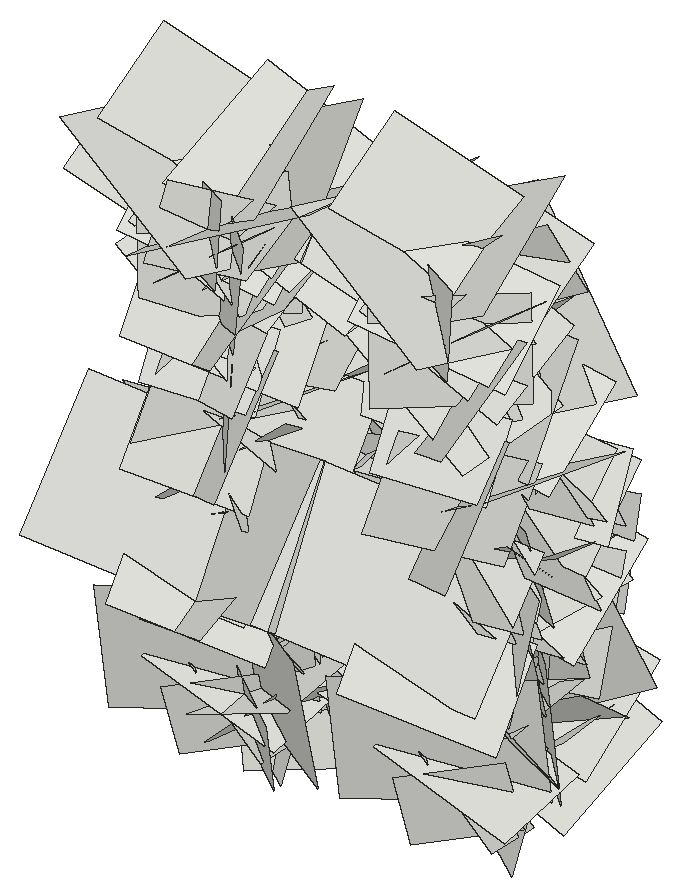
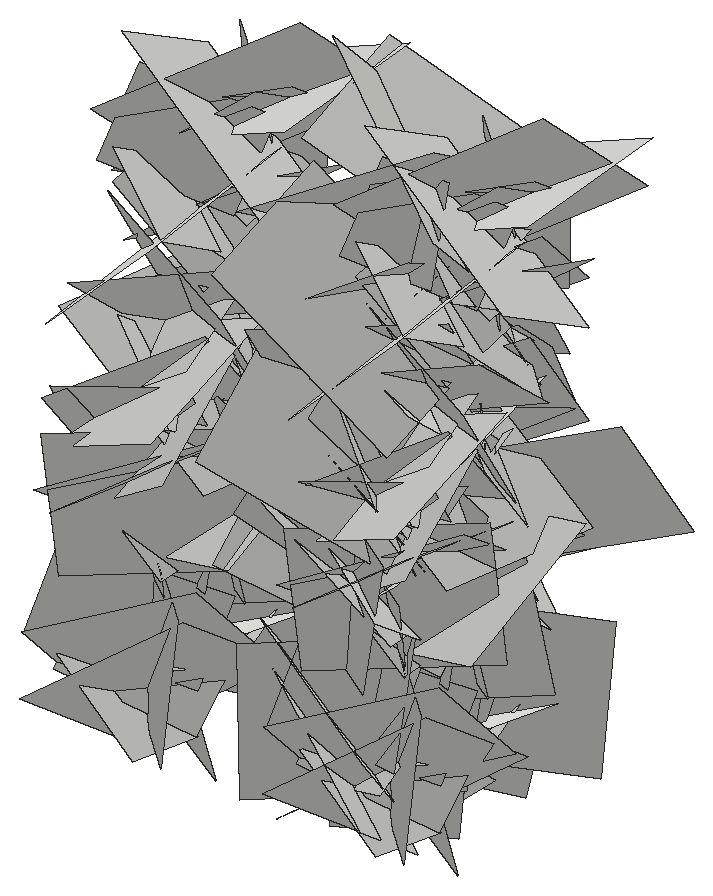
# SketchUp Ruby script. Lengths in inches.
U = 1.inch
M = Sketchup.active_model
def pt(a) = Geom::Point3d.new(a.map { |v| v * U })
def face(e, loops, mat)
  f = e.add_face(loops[0].map { |a| pt(a) })
  loops[1..].each { |l| e.add_face(l.map { |a| pt(a) }).erase! }
  f.material = f.back_material = mat if mat
  f
end
# faces: each face lists its corners as indices into pts; further lists are holes
def faces(e, pts, list, mat = nil) = list.each { |f| face(e, (f[0].is_a?(Array) ? f : [f]).map { |l| l.map { |i| pts[i] } }, mat) }
# xy, xz, yz: faces in a plane at the given z, y or x. An outline is a flat list of corners, or four numbers for a rectangle; further outlines are holes
def ring(l) = l.size == 4 ? [[l[0], l[1]], [l[2], l[1]], [l[2], l[3]], [l[0], l[3]]] : l.each_slice(2).to_a
def flat(e, list, mat, &to3) = list.each { |f| face(e, (f[0].is_a?(Array) ? f : [f]).map { |l| ring(l).map { |u, v| to3.(u, v) } }, mat) }
def xy(e, z, list, mat = nil) = flat(e, list, mat) { |x, y| [x, y, z] }
def xz(e, y, list, mat = nil) = flat(e, list, mat) { |x, z| [x, y, z] }
def yz(e, x, list, mat = nil) = flat(e, list, mat) { |y, z| [x, y, z] }
def lines(e, pts, list) = list.each { |a, b| e.add_line(pt(pts[a]), pt(pts[b])) }
# prism: a flat outline (further loops are holes) pulled along v
def prism(e, loops, v, mat = nil)
  f = face(e, loops, mat); d = Geom::Vector3d.new(v.map { |x| x * U })
  f.pushpull(f.normal.samedirection?(d) ? d.length : -d.length)
end
def box(e, o, s, mat = nil) = prism(e, [[o, [o[0] + s[0], o[1], o[2]], [o[0] + s[0], o[1] + s[1], o[2]], [o[0], o[1] + s[1], o[2]]]], [0, 0, s[2]], mat)
def at(x, y, z, deg = 0) = Geom::Transformation.translation(pt([x, y, z])) * Geom::Transformation.rotation(ORIGIN, Z_AXIS, deg.degrees)
def axes(o, x, y, z) = Geom::Transformation.new([*x, 0, *y, 0, *z, 0, *pt(o).to_a, 1])
def part(name) = M.definitions.add(name)
# library, detail: a bought-in or finely detailed component or shape, given as its bounding box
def library(name, o, s) = part(name).tap { |d| box(d.entities, o, s) }
def detail(e, o, s) = box(e.add_group.entities, o, s)
def put(e, d, t, mat = nil) = e.add_instance(d, t).tap { |i| i.material = mat if mat }
def group(e, t, mat = nil) = e.add_group.tap { |g| g.transformation = t; g.material = mat if mat }.entities
root = M.entities
c1 = part("Component\#6")
p = [[0.01,0,0],[0,3.24,4.54],[4.32,3.24,4.54],[4.33,0,0]]
faces(c1.entities,p,[[0,1,2,3]])
put(root,c1,axes([404.88,177.17,11.87],[-0.09089,-0.73345,-1.16692],[-0.11565,-1.16189,0.73831],[-1.45639,0.13804,0.0142]))
put(root,c1,axes([400.91,177.17,11.87],[0.09089,-0.73345,-1.16692],[0.11565,-1.16189,0.73831],[1.45639,0.13804,0.0142]))
put(root,c1,axes([414.68,177.17,11.87],[-0.09089,-0.73345,-1.16692],[-0.11565,-1.16189,0.73831],[-1.45639,0.13804,0.0142]))
put(root,c1,axes([400.91,171.15,7.72],[-0.19789,0.75168,0.59634],[0.00491,0.60823,-0.76521],[1.01706,0.14332,0.11972]))
put(root,c1,axes([404.88,171.15,7.72],[0.19789,0.75168,0.59634],[-0.00491,0.60823,-0.76521],[-1.01706,0.14332,0.11972]))
put(root,c1,axes([410.71,171.15,7.72],[-0.19789,0.75168,0.59634],[0.00491,0.60823,-0.76521],[1.01706,0.14332,0.11972]))
put(root,c1,axes([400.91,175.79,22.11],[0.09057,-0.18477,-0.67682],[-0.07729,-0.68047,0.17656],[0.73966,-0.04848,0.10132]))
put(root,c1,axes([404.88,175.79,22.11],[-0.09057,-0.18477,-0.67682],[0.07729,-0.68047,0.17656],[-0.73966,-0.04848,0.10132]))
put(root,c1,axes([410.71,175.79,22.11],[0.09057,-0.18477,-0.67682],[-0.07729,-0.68047,0.17656],[0.73966,-0.04848,0.10132]))
put(root,c1,axes([400.91,172.87,15.39],[-0.04258,0.36909,0.59744],[0.18529,0.58484,-0.34955],[0.72096,-0.1285,0.12512]))
put(root,c1,axes([404.88,172.87,15.39],[0.04258,0.36909,0.59744],[-0.18529,0.58484,-0.34955],[-0.72096,-0.1285,0.12512]))
put(root,c1,axes([410.71,172.87,15.39],[-0.04258,0.36909,0.59744],[0.18529,0.58484,-0.34955],[0.72096,-0.1285,0.12512]))
put(root,c1,axes([404.88,176.71,20],[-0.1716,-1.2405,0.25629],[-0.15029,0.2745,1.23906],[-1.33426,0.12862,-0.17253]))
put(root,c1,axes([400.91,176.71,20],[0.1716,-1.2405,0.25629],[0.15029,0.2745,1.23906],[1.33426,0.12862,-0.17253]))
put(root,c1,axes([414.68,176.71,20],[-0.1716,-1.2405,0.25629],[-0.15029,0.2745,1.23906],[-1.33426,0.12862,-0.17253]))
put(root,c1,axes([400.91,172.9,17.79],[-0.05847,0.04666,0.93522],[-0.13105,0.92828,-0.05361],[0.98388,0.12642,0.04844]))
put(root,c1,axes([404.88,172.9,17.79],[0.05847,0.04666,0.93522],[0.13105,0.92828,-0.05361],[-0.98388,0.12642,0.04844]))
put(root,c1,axes([410.71,172.9,17.79],[-0.05847,0.04666,0.93522],[-0.13105,0.92828,-0.05361],[0.98388,0.12642,0.04844]))
put(root,c1,axes([400.91,172.44,13.26],[0.14239,0.27787,0.83247],[-0.25689,0.82117,-0.23499],[0.89411,0.19168,-0.20009]))
put(root,c1,axes([404.88,172.44,13.26],[-0.14239,0.27787,0.83247],[0.25689,0.82117,-0.23499],[-0.89411,0.19168,-0.20009]))
put(root,c1,axes([410.71,172.44,13.26],[0.14239,0.27787,0.83247],[-0.25689,0.82117,-0.23499],[0.89411,0.19168,-0.20009]))
put(root,c1,axes([400.91,178.76,18.36],[-0.19902,-0.79911,-0.76231],[-0.1591,-0.74761,0.82067],[1.1598,-0.23968,-0.01823]))
put(root,c1,axes([404.88,178.76,18.36],[0.19902,-0.79911,-0.76231],[0.1591,-0.74761,0.82067],[-1.1598,-0.23968,-0.01823]))
put(root,c1,axes([410.71,178.76,18.36],[-0.19902,-0.79911,-0.76231],[-0.1591,-0.74761,0.82067],[1.1598,-0.23968,-0.01823]))
put(root,c1,axes([404.88,178.02,21.625],[0.10055,-0.80704,-0.57155],[-0.14009,-0.57937,0.79615],[-1.03886,0.00001,-0.16268]))
put(root,c1,axes([400.91,178.02,21.625],[-0.10055,-0.80704,-0.57155],[0.14009,-0.57937,0.79615],[1.03886,0.00001,-0.16268]))
put(root,c1,axes([414.68,178.02,21.625],[0.10055,-0.80704,-0.57155],[-0.14009,-0.57937,0.79615],[-1.03886,0.00001,-0.16268]))
put(root,c1,axes([404.88,171.875,12.53],[0.03767,0.74177,1.03266],[0.14299,1.02503,-0.74093],[-1.34014,0.13022,-0.05004]))
put(root,c1,axes([400.91,171.875,12.53],[-0.03767,0.74177,1.03266],[-0.14299,1.02503,-0.74093],[1.34014,0.13022,-0.05004]))
put(root,c1,axes([414.68,171.875,12.53],[0.03767,0.74177,1.03266],[0.14299,1.02503,-0.74093],[-1.34014,0.13022,-0.05004]))
put(root,c1,axes([400.91,176.92,18.36],[0.03591,-0.7978,0.13647],[-0.05211,0.13431,0.79737],[0.85636,0.04162,0.0428]))
put(root,c1,axes([404.88,176.92,18.36],[-0.03591,-0.7978,0.13647],[0.05211,0.13431,0.79737],[-0.85636,0.04162,0.0428]))
put(root,c1,axes([410.71,176.92,18.36],[0.03591,-0.7978,0.13647],[-0.05211,0.13431,0.79737],[0.85636,0.04162,0.0428]))
put(root,c1,axes([404.88,176.79,7.17],[-0.05072,0.23896,-1.1979],[-0.10512,-1.19562,-0.23454],[-1.29052,0.088,0.06618]))
put(root,c1,axes([400.91,176.79,7.17],[0.05072,0.23896,-1.1979],[0.10512,-1.19562,-0.23454],[1.29052,0.088,0.06618]))
put(root,c1,axes([414.68,176.79,7.17],[-0.05072,0.23896,-1.1979],[-0.10512,-1.19562,-0.23454],[-1.29052,0.088,0.06618]))
put(root,c1,axes([400.91,175.07,0.3],[-0.05353,-0.16234,0.63718],[-0.01427,0.63917,0.16178],[0.69684,0.00062,0.05226]))
put(root,c1,axes([404.88,175.07,0.3],[0.05353,-0.16234,0.63718],[0.01427,0.63917,0.16178],[-0.69684,0.00062,0.05226]))
put(root,c1,axes([410.71,175.07,0.3],[-0.05353,-0.16234,0.63718],[-0.01427,0.63917,0.16178],[0.69684,0.00062,0.05226]))
put(root,c1,axes([404.88,178.16,17.01],[-0.17232,-1.0163,-0.23365],[0.0611,-0.24487,1.02499],[-1.10369,0.14512,0.09322]))
put(root,c1,axes([400.91,178.16,17.01],[0.17232,-1.0163,-0.23365],[-0.0611,-0.24487,1.02499],[1.10369,0.14512,0.09322]))
put(root,c1,axes([414.68,178.16,17.01],[-0.17232,-1.0163,-0.23365],[0.0611,-0.24487,1.02499],[-1.10369,0.14512,0.09322]))
put(root,c1,axes([404.88,178.75,19.8],[-0.0392,-0.90326,-0.49419],[0.16181,-0.49385,0.89122],[-1.07932,-0.04123,0.15156]))
put(root,c1,axes([400.91,178.75,19.8],[0.0392,-0.90326,-0.49419],[-0.16181,-0.49385,0.89122],[1.07932,-0.04123,0.15156]))
put(root,c1,axes([414.68,178.75,19.8],[-0.0392,-0.90326,-0.49419],[0.16181,-0.49385,0.89122],[-1.07932,-0.04123,0.15156]))
put(root,c1,axes([400.91,174.43,8.39],[-0.03188,0.26889,0.69876],[0.00311,0.69936,-0.269],[0.79363,0.00806,0.02912]))
put(root,c1,axes([404.88,174.43,8.39],[0.03188,0.26889,0.69876],[-0.00311,0.69936,-0.269],[-0.79363,0.00806,0.02912]))
put(root,c1,axes([410.71,174.43,8.39],[-0.03188,0.26889,0.69876],[0.00311,0.69936,-0.269],[0.79363,0.00806,0.02912]))
put(root,c1,axes([404.88,179.79,22.45],[-0.18749,-0.99323,-0.93091],[0.09936,-0.94539,0.99088],[-1.43954,0.06411,0.18963]))
put(root,c1,axes([400.91,179.79,22.45],[0.18749,-0.99323,-0.93091],[-0.09936,-0.94539,0.99088],[1.43954,0.06411,0.18963]))
put(root,c1,axes([414.68,179.79,22.45],[-0.18749,-0.99323,-0.93091],[0.09936,-0.94539,0.99088],[-1.43954,0.06411,0.18963]))
put(root,c1,axes([404.88,177.03,8.61],[-0.03763,-0.79919,0.49947],[0.19388,0.48448,0.78821],[-0.97999,0.12653,0.13676]))
put(root,c1,axes([400.91,177.03,8.61],[0.03763,-0.79919,0.49947],[-0.19388,0.48448,0.78821],[0.97999,0.12653,0.13676]))
put(root,c1,axes([414.68,177.03,8.61],[-0.03763,-0.79919,0.49947],[0.19388,0.48448,0.78821],[-0.97999,0.12653,0.13676]))
put(root,c1,axes([400.91,177.03,9.04],[-0.05145,-0.49737,0.47013],[0.11624,0.45957,0.49752],[0.71609,-0.11034,-0.04698]))
put(root,c1,axes([404.88,177.03,9.04],[0.05145,-0.49737,0.47013],[-0.11624,0.45957,0.49752],[-0.71609,-0.11034,-0.04698]))
put(root,c1,axes([410.71,177.03,9.04],[-0.05145,-0.49737,0.47013],[0.11624,0.45957,0.49752],[0.71609,-0.11034,-0.04698]))
put(root,c1,axes([404.88,179.02,2.63],[0.02304,-0.93672,-0.18796],[-0.20199,-0.18848,0.91728],[-0.99236,0.01662,-0.19107]))
put(root,c1,axes([400.91,179.02,2.63],[-0.02304,-0.93672,-0.18796],[0.20199,-0.18848,0.91728],[0.99236,0.01662,-0.19107]))
put(root,c1,axes([414.68,179.02,2.63],[0.02304,-0.93672,-0.18796],[-0.20199,-0.18848,0.91728],[-0.99236,0.01662,-0.19107]))
put(root,c1,axes([400.91,175.31,3.87],[-0.17194,0.72285,-0.14796],[-0.1038,-0.17124,-0.72925],[0.77519,0.1374,-0.13047]))
put(root,c1,axes([404.88,175.31,3.87],[0.17194,0.72285,-0.14796],[0.1038,-0.17124,-0.72925],[-0.77519,0.1374,-0.13047]))
put(root,c1,axes([410.71,175.31,3.87],[-0.17194,0.72285,-0.14796],[-0.1038,-0.17124,-0.72925],[0.77519,0.1374,-0.13047]))
put(root,c1,axes([404.88,173.88,22.27],[-0.13701,1.18016,0.66561],[-0.07419,0.66193,-1.18721],[-1.4343,-0.14697,-0.00217]))
put(root,c1,axes([400.91,173.88,22.27],[0.13701,1.18016,0.66561],[0.07419,0.66193,-1.18721],[1.4343,-0.14697,-0.00217]))
put(root,c1,axes([414.68,173.88,22.27],[-0.13701,1.18016,0.66561],[-0.07419,0.66193,-1.18721],[-1.4343,-0.14697,-0.00217]))
put(root,c1,axes([404.88,175.28,5.97],[0.1544,0.17587,1.10387],[-0.02973,1.11343,-0.17369],[-1.18449,-0.00502,0.14825]))
put(root,c1,axes([400.91,175.28,5.97],[-0.1544,0.17587,1.10387],[0.02973,1.11343,-0.17369],[1.18449,-0.00502,0.14825]))
put(root,c1,axes([414.68,175.28,5.97],[0.1544,0.17587,1.10387],[-0.02973,1.11343,-0.17369],[-1.18449,-0.00502,0.14825]))
put(root,c1,axes([404.88,174.05,15.13],[0.29087,1.34123,-0.04275],[-0.1118,-0.02194,-1.36543],[-1.41802,0.27684,0.09888]))
put(root,c1,axes([400.91,174.05,15.13],[-0.29087,1.34123,-0.04275],[0.1118,-0.02194,-1.36543],[1.41802,0.27684,0.09888]))
put(root,c1,axes([414.68,174.05,15.13],[0.29087,1.34123,-0.04275],[-0.1118,-0.02194,-1.36543],[-1.41802,0.27684,0.09888]))
put(root,c1,axes([404.88,177.91,2.6],[-0.0759,-0.493,0.60539],[-0.11612,0.60826,0.48238],[-0.8194,-0.04053,-0.12444]))
put(root,c1,axes([400.91,177.91,2.6],[0.0759,-0.493,0.60539],[0.11612,0.60826,0.48238],[0.8194,-0.04053,-0.12444]))
put(root,c1,axes([414.68,177.91,2.6],[-0.0759,-0.493,0.60539],[-0.11612,0.60826,0.48238],[-0.8194,-0.04053,-0.12444]))
put(root,c1,axes([400.91,179.07,16.9375],[0.01654,-0.76992,0.15337],[-0.18248,0.14631,0.752],[0.8119,0.04857,0.16589]))
put(root,c1,axes([404.88,179.07,16.9375],[-0.01654,-0.76992,0.15337],[0.18248,0.14631,0.752],[-0.8119,0.04857,0.16589]))
put(root,c1,axes([410.71,179.07,16.9375],[0.01654,-0.76992,0.15337],[-0.18248,0.14631,0.752],[0.8119,0.04857,0.16589]))
put(root,c1,axes([404.88,177.25,5.58],[-0.00826,-0.19404,0.73725],[-0.12542,0.72866,0.19053],[-0.79831,-0.11247,-0.03756]))
put(root,c1,axes([400.91,177.25,5.58],[0.00826,-0.19404,0.73725],[0.12542,0.72866,0.19053],[0.79831,-0.11247,-0.03756]))
put(root,c1,axes([414.68,177.25,5.58],[-0.00826,-0.19404,0.73725],[-0.12542,0.72866,0.19053],[-0.79831,-0.11247,-0.03756]))
put(root,c1,axes([400.91,178.9,4.98],[-0.12785,-0.58421,0.25103],[0.01096,0.25367,0.59532],[0.67392,-0.11496,0.03794]))
put(root,c1,axes([404.88,178.9,4.98],[0.12785,-0.58421,0.25103],[-0.01096,0.25367,0.59532],[-0.67392,-0.11496,0.03794]))
put(root,c1,axes([410.71,178.9,4.98],[-0.12785,-0.58421,0.25103],[0.01096,0.25367,0.59532],[0.67392,-0.11496,0.03794]))
put(root,c1,axes([400.91,177.55,19],[-0.11507,-0.3549,0.71119],[-0.00206,0.71791,0.35796],[0.84251,-0.04671,0.09801]))
put(root,c1,axes([404.88,177.55,19],[0.11507,-0.3549,0.71119],[0.00206,0.71791,0.35796],[-0.84251,-0.04671,0.09801]))
put(root,c1,axes([410.71,177.55,19],[-0.11507,-0.3549,0.71119],[-0.00206,0.71791,0.35796],[0.84251,-0.04671,0.09801]))
put(root,c1,axes([404.88,179.43,6.59],[-0.14458,-1.15784,0.73248],[-0.20973,0.74503,1.14083],[-1.43706,0.00775,-0.24019]))
put(root,c1,axes([400.91,179.43,6.59],[0.14458,-1.15784,0.73248],[0.20973,0.74503,1.14083],[1.43706,0.00775,-0.24019]))
put(root,c1,axes([414.68,179.43,6.59],[-0.14458,-1.15784,0.73248],[-0.20973,0.74503,1.14083],[-1.43706,0.00775,-0.24019]))
put(root,c1,axes([404.88,177.67,8.79],[-0.10774,-0.22129,0.90038],[-0.20078,0.89162,0.19775],[-0.96207,-0.1613,-0.1421]))
put(root,c1,axes([400.91,177.67,8.79],[0.10774,-0.22129,0.90038],[0.20078,0.89162,0.19775],[0.96207,-0.1613,-0.1421]))
put(root,c1,axes([414.68,177.67,8.79],[-0.10774,-0.22129,0.90038],[-0.20078,0.89162,0.19775],[-0.96207,-0.1613,-0.1421]))
put(root,c1,axes([400.91,179.66,2.51],[-0.14219,-0.09473,-0.68692],[0.01318,-0.69988,0.09409],[0.73491,-0.00578,-0.13459]))
put(root,c1,axes([404.88,179.66,2.51],[0.14219,-0.09473,-0.68692],[-0.01318,-0.69988,0.09409],[-0.73491,-0.00578,-0.13459]))
put(root,c1,axes([410.71,179.66,2.51],[-0.14219,-0.09473,-0.68692],[0.01318,-0.69988,0.09409],[0.73491,-0.00578,-0.13459]))
put(root,c1,axes([400.91,180.59,3.91],[-0.10883,-0.74668,-0.23347],[0.0349,-0.23939,0.75113],[0.82853,-0.08799,-0.06231]))
put(root,c1,axes([404.88,180.59,3.91],[0.10883,-0.74668,-0.23347],[-0.0349,-0.23939,0.75113],[-0.82853,-0.08799,-0.06231]))
put(root,c1,axes([410.71,180.59,3.91],[-0.10883,-0.74668,-0.23347],[0.0349,-0.23939,0.75113],[0.82853,-0.08799,-0.06231]))
put(root,c1,axes([400.91,180.83,12.7],[-0.12371,-0.65209,-0.45157],[-0.04757,-0.45027,0.66181],[0.83942,-0.12162,-0.02905]))
put(root,c1,axes([404.88,180.83,12.7],[0.12371,-0.65209,-0.45157],[0.04757,-0.45027,0.66181],[-0.83942,-0.12162,-0.02905]))
put(root,c1,axes([410.71,180.83,12.7],[-0.12371,-0.65209,-0.45157],[-0.04757,-0.45027,0.66181],[0.83942,-0.12162,-0.02905]))
put(root,c1,axes([404.88,180.99,16.6875],[-0.01817,-0.80344,-0.66577],[-0.22863,-0.64876,0.78846],[-1.08217,0.15055,-0.1554]))
put(root,c1,axes([400.91,180.99,16.6875],[0.01817,-0.80344,-0.66577],[0.22863,-0.64876,0.78846],[1.08217,0.15055,-0.1554]))
put(root,c1,axes([414.68,180.99,16.6875],[-0.01817,-0.80344,-0.66577],[-0.22863,-0.64876,0.78846],[-1.08217,0.15055,-0.1554]))
put(root,c1,axes([404.88,176.29,14.82],[-0.00549,0.62123,1.00169],[-0.24363,0.98194,-0.61017],[-1.22543,-0.19801,0.11682]))
put(root,c1,axes([400.91,176.29,14.82],[0.00549,0.62123,1.00169],[0.24363,0.98194,-0.61017],[1.22543,-0.19801,0.11682]))
put(root,c1,axes([414.68,176.29,14.82],[-0.00549,0.62123,1.00169],[-0.24363,0.98194,-0.61017],[-1.22543,-0.19801,0.11682]))
put(root,c1,axes([400.91,178.54,4.68],[0.06155,-0.26232,0.60589],[0.0363,0.6086,0.26022],[0.69891,-0.00851,-0.06687]))
put(root,c1,axes([404.88,178.54,4.68],[-0.06155,-0.26232,0.60589],[-0.0363,0.6086,0.26022],[-0.69891,-0.00851,-0.06687]))
put(root,c1,axes([410.71,178.54,4.68],[0.06155,-0.26232,0.60589],[0.0363,0.6086,0.26022],[0.69891,-0.00851,-0.06687]))
put(root,c1,axes([404.88,179.8125,11.71],[-0.00414,-0.7832,0.49624],[0.01003,0.49619,0.78318],[-0.98275,0.00836,0.0059]))
put(root,c1,axes([414.68,179.8125,11.71],[-0.00414,-0.7832,0.49624],[0.01003,0.49619,0.78318],[-0.98275,0.00836,0.0059]))
put(root,c1,axes([400.91,179.8125,11.71],[0.00414,-0.7832,0.49624],[-0.01003,0.49619,0.78318],[0.98275,0.00836,0.0059]))
put(root,c1,axes([404.88,181.49,10.05],[-0.07357,-0.24485,-1.22332],[-0.09578,-1.221,0.24951],[-1.31896,0.10233,0.05011]))
put(root,c1,axes([400.91,181.49,10.05],[0.07357,-0.24485,-1.22332],[0.09578,-1.221,0.24951],[1.31896,0.10233,0.05011]))
put(root,c1,axes([414.68,181.49,10.05],[-0.07357,-0.24485,-1.22332],[-0.09578,-1.221,0.24951],[-1.31896,0.10233,0.05011]))
put(root,c1,axes([400.91,181.21,19.66],[-0.0984,-0.57654,-0.29954],[-0.01889,-0.30021,0.58335],[0.68843,-0.09064,-0.02681]))
put(root,c1,axes([404.88,181.21,19.66],[0.0984,-0.57654,-0.29954],[0.01889,-0.30021,0.58335],[-0.68843,-0.09064,-0.02681]))
put(root,c1,axes([410.71,181.21,19.66],[-0.0984,-0.57654,-0.29954],[-0.01889,-0.30021,0.58335],[0.68843,-0.09064,-0.02681]))
put(root,c1,axes([400.91,181.24,7.39],[-0.09835,-0.8461,0.11424],[-0.10744,0.12502,0.84359],[0.89861,-0.07766,0.11336]))
put(root,c1,axes([404.88,181.24,7.39],[0.09835,-0.8461,0.11424],[0.10744,0.12502,0.84359],[-0.89861,-0.07766,0.11336]))
put(root,c1,axes([410.71,181.24,7.39],[-0.09835,-0.8461,0.11424],[-0.10744,0.12502,0.84359],[0.89861,-0.07766,0.11336]))
put(root,c1,axes([404.88,180.26,8.26],[0.04265,-1.00211,0.75475],[0.17142,0.75298,0.99114],[-1.31872,0.06547,0.15325]))
put(root,c1,axes([400.91,180.26,8.26],[-0.04265,-1.00211,0.75475],[-0.17142,0.75298,0.99114],[1.31872,0.06547,0.15325]))
put(root,c1,axes([414.68,180.26,8.26],[0.04265,-1.00211,0.75475],[0.17142,0.75298,0.99114],[-1.31872,0.06547,0.15325]))
put(root,c1,axes([404.88,182.69,9.96],[0.0402,-0.96504,-0.67279],[-0.04089,-0.67379,0.96431],[-1.24632,-0.00902,-0.05333]))
put(root,c1,axes([400.91,182.69,9.96],[-0.0402,-0.96504,-0.67279],[0.04089,-0.67379,0.96431],[1.24632,-0.00902,-0.05333]))
put(root,c1,axes([414.68,182.69,9.96],[0.0402,-0.96504,-0.67279],[-0.04089,-0.67379,0.96431],[-1.24632,-0.00902,-0.05333]))
put(root,c1,axes([404.88,182.3,13.14],[-0.06012,-0.59744,-0.78978],[0.12867,-0.78931,0.58836],[-1.0418,-0.06301,0.11824]))
put(root,c1,axes([400.91,182.3,13.14],[0.06012,-0.59744,-0.78978],[-0.12867,-0.78931,0.58836],[1.0418,-0.06301,0.11824]))
put(root,c1,axes([414.68,182.3,13.14],[-0.06012,-0.59744,-0.78978],[0.12867,-0.78931,0.58836],[-1.0418,-0.06301,0.11824]))
put(root,c1,axes([400.91,181.23,7.68],[0.09173,-0.20092,-0.6203],[-0.07215,-0.6251,0.19298],[0.68737,-0.0388,0.10304]))
put(root,c1,axes([404.88,181.23,7.68],[-0.09173,-0.20092,-0.6203],[0.07215,-0.6251,0.19298],[-0.68737,-0.0388,0.10304]))
put(root,c1,axes([410.71,181.23,7.68],[0.09173,-0.20092,-0.6203],[-0.07215,-0.6251,0.19298],[0.68737,-0.0388,0.10304]))
put(root,c1,axes([404.88,179.12,5.58],[-0.07323,0.67973,-0.51678],[-0.08286,-0.52133,-0.67526],[-0.90131,-0.0073,0.10406]))
put(root,c1,axes([400.91,179.12,5.58],[0.07323,0.67973,-0.51678],[0.08286,-0.52133,-0.67526],[0.90131,-0.0073,0.10406]))
put(root,c1,axes([414.68,179.12,5.58],[-0.07323,0.67973,-0.51678],[-0.08286,-0.52133,-0.67526],[-0.90131,-0.0073,0.10406]))
put(root,c1,axes([404.88,181.89,8.77],[-0.15486,-1.04414,-0.08659],[0.04063,-0.0927,1.0531],[-1.10985,0.1423,0.05063]))
put(root,c1,axes([400.91,181.89,8.77],[0.15486,-1.04414,-0.08659],[-0.04063,-0.0927,1.0531],[1.10985,0.1423,0.05063]))
put(root,c1,axes([414.68,181.89,8.77],[-0.15486,-1.04414,-0.08659],[0.04063,-0.0927,1.0531],[-1.10985,0.1423,0.05063]))
put(root,c1,axes([404.88,182.08,15.67],[-0.13861,-1.35642,0.31459],[0.2886,0.28497,1.34186],[-1.44748,0.1867,0.23742]))
put(root,c1,axes([400.91,182.08,15.67],[0.13861,-1.35642,0.31459],[-0.2886,0.28497,1.34186],[1.44748,0.1867,0.23742]))
put(root,c1,axes([414.68,182.08,15.67],[-0.13861,-1.35642,0.31459],[0.2886,0.28497,1.34186],[-1.44748,0.1867,0.23742]))
put(root,c1,axes([404.88,180.69,8.55],[0.12889,0.40226,-0.91097],[0.04748,-0.91901,-0.39983],[-1.05451,0.00779,-0.12935]))
put(root,c1,axes([414.68,180.69,8.55],[0.12889,0.40226,-0.91097],[0.04748,-0.91901,-0.39983],[-1.05451,0.00779,-0.12935]))
put(root,c1,axes([400.91,180.69,8.55],[-0.12889,0.40226,-0.91097],[-0.04748,-0.91901,-0.39983],[1.05451,0.00779,-0.12935]))
put(root,c1,axes([404.88,178.03,1.86],[-0.09591,-0.07879,1.2407],[0.19288,1.22975,0.09137],[-1.3036,0.18775,-0.07776]))
put(root,c1,axes([400.91,178.03,1.86],[0.09591,-0.07879,1.2407],[-0.19288,1.22975,0.09137],[1.3036,0.18775,-0.07776]))
put(root,c1,axes([414.68,178.03,1.86],[-0.09591,-0.07879,1.2407],[0.19288,1.22975,0.09137],[-1.3036,0.18775,-0.07776]))
put(root,c1,axes([400.91,178.57,11.38],[-0.09025,0.42259,0.64735],[0.15778,0.64804,-0.40347],[0.80413,-0.07973,0.15182]))
put(root,c1,axes([404.88,178.57,11.38],[0.09025,0.42259,0.64735],[-0.15778,0.64804,-0.40347],[-0.80413,-0.07973,0.15182]))
put(root,c1,axes([410.71,178.57,11.38],[-0.09025,0.42259,0.64735],[0.15778,0.64804,-0.40347],[0.80413,-0.07973,0.15182]))
put(root,c1,axes([404.88,181.48,10.98],[-0.16941,-1.10786,0.62997],[0.04307,0.63015,1.11849],[-1.35023,0.1591,-0.04336]))
put(root,c1,axes([400.91,181.48,10.98],[0.16941,-1.10786,0.62997],[-0.04307,0.63015,1.11849],[1.35023,0.1591,-0.04336]))
put(root,c1,axes([414.68,181.48,10.98],[-0.16941,-1.10786,0.62997],[0.04307,0.63015,1.11849],[-1.35023,0.1591,-0.04336]))
put(root,c1,axes([404.88,183.39,2.71],[-0.21072,-0.93049,-0.66529],[0.0846,-0.6849,0.93407],[-1.20954,0.1142,0.18123]))
put(root,c1,axes([400.91,183.39,2.71],[0.21072,-0.93049,-0.66529],[-0.0846,-0.6849,0.93407],[1.20954,0.1142,0.18123]))
put(root,c1,axes([414.68,183.39,2.71],[-0.21072,-0.93049,-0.66529],[0.0846,-0.6849,0.93407],[-1.20954,0.1142,0.18123]))
put(root,c1,axes([404.88,182.3,11.84],[-0.17648,0.01407,-1.1199],[-0.09677,-1.12861,-0.00061],[-1.18323,0.09021,0.16708]))
put(root,c1,axes([400.91,182.3,11.84],[0.17648,0.01407,-1.1199],[0.09677,-1.12861,-0.00061],[1.18323,0.09021,0.16708]))
put(root,c1,axes([414.68,182.3,11.84],[-0.17648,0.01407,-1.1199],[-0.09677,-1.12861,-0.00061],[-1.18323,0.09021,0.16708]))
put(root,c1,axes([404.88,183.3125,5.12],[-0.15127,-0.71846,-0.81538],[-0.11003,-0.80961,0.73154],[-1.14669,0.17246,0.03737]))
put(root,c1,axes([400.91,183.3125,5.12],[0.15127,-0.71846,-0.81538],[0.11003,-0.80961,0.73154],[1.14669,0.17246,0.03737]))
put(root,c1,axes([414.68,183.3125,5.12],[-0.15127,-0.71846,-0.81538],[-0.11003,-0.80961,0.73154],[-1.14669,0.17246,0.03737]))
put(root,c1,axes([400.91,182.67,1.51],[-0.02969,-0.72745,-0.10184],[-0.03667,-0.1005,0.72735],[0.77775,-0.03251,0.03041]))
put(root,c1,axes([404.88,182.67,1.51],[0.02969,-0.72745,-0.10184],[0.03667,-0.1005,0.72735],[-0.77775,-0.03251,0.03041]))
put(root,c1,axes([410.71,182.67,1.51],[-0.02969,-0.72745,-0.10184],[-0.03667,-0.1005,0.72735],[0.77775,-0.03251,0.03041]))
